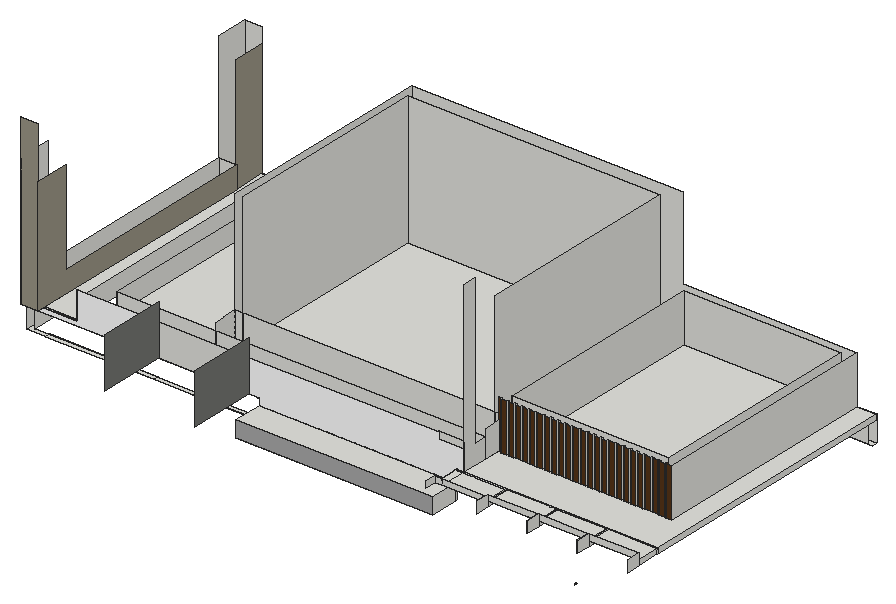
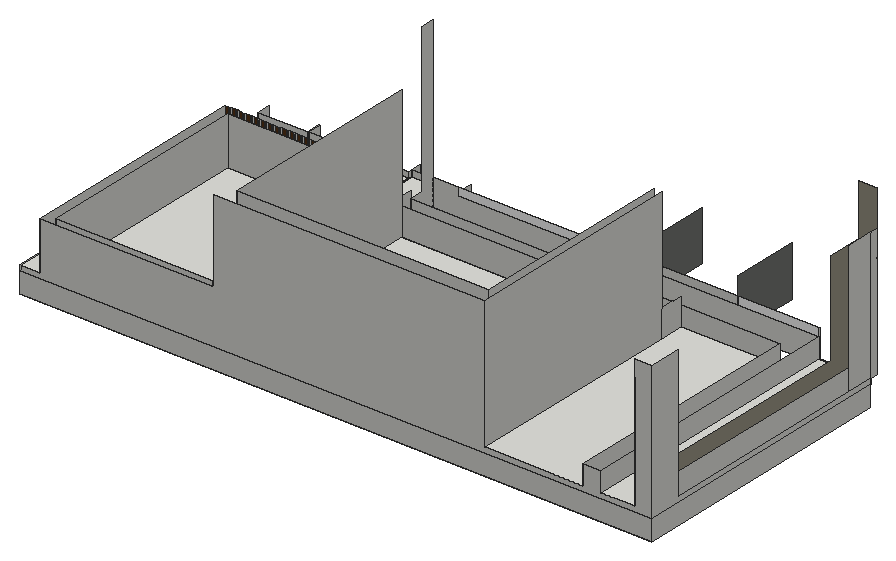
# SketchUp Ruby script. Lengths in inches.
U = 1.inch
M = Sketchup.active_model
def pt(a) = Geom::Point3d.new(a.map { |v| v * U })
def face(e, loops, mat)
  f = e.add_face(loops[0].map { |a| pt(a) })
  loops[1..].each { |l| e.add_face(l.map { |a| pt(a) }).erase! }
  f.material = f.back_material = mat if mat
  f
end
# faces: each face lists its corners as indices into pts; further lists are holes
def faces(e, pts, list, mat = nil) = list.each { |f| face(e, (f[0].is_a?(Array) ? f : [f]).map { |l| l.map { |i| pts[i] } }, mat) }
# xy, xz, yz: faces in a plane at the given z, y or x. An outline is a flat list of corners, or four numbers for a rectangle; further outlines are holes
def ring(l) = l.size == 4 ? [[l[0], l[1]], [l[2], l[1]], [l[2], l[3]], [l[0], l[3]]] : l.each_slice(2).to_a
def flat(e, list, mat, &to3) = list.each { |f| face(e, (f[0].is_a?(Array) ? f : [f]).map { |l| ring(l).map { |u, v| to3.(u, v) } }, mat) }
def xy(e, z, list, mat = nil) = flat(e, list, mat) { |x, y| [x, y, z] }
def xz(e, y, list, mat = nil) = flat(e, list, mat) { |x, z| [x, y, z] }
def yz(e, x, list, mat = nil) = flat(e, list, mat) { |y, z| [x, y, z] }
def lines(e, pts, list) = list.each { |a, b| e.add_line(pt(pts[a]), pt(pts[b])) }
# prism: a flat outline (further loops are holes) pulled along v
def prism(e, loops, v, mat = nil)
  f = face(e, loops, mat); d = Geom::Vector3d.new(v.map { |x| x * U })
  f.pushpull(f.normal.samedirection?(d) ? d.length : -d.length)
end
def box(e, o, s, mat = nil) = prism(e, [[o, [o[0] + s[0], o[1], o[2]], [o[0] + s[0], o[1] + s[1], o[2]], [o[0], o[1] + s[1], o[2]]]], [0, 0, s[2]], mat)
def at(x, y, z, deg = 0) = Geom::Transformation.translation(pt([x, y, z])) * Geom::Transformation.rotation(ORIGIN, Z_AXIS, deg.degrees)
def axes(o, x, y, z) = Geom::Transformation.new([*x, 0, *y, 0, *z, 0, *pt(o).to_a, 1])
def part(name) = M.definitions.add(name)
# library, detail: a bought-in or finely detailed component or shape, given as its bounding box
def library(name, o, s) = part(name).tap { |d| box(d.entities, o, s) }
def detail(e, o, s) = box(e.add_group.entities, o, s)
def put(e, d, t, mat = nil) = e.add_instance(d, t).tap { |i| i.material = mat if mat }
def group(e, t, mat = nil) = e.add_group.tap { |g| g.transformation = t; g.material = mat if mat }.entities
root = M.entities
M.materials.add("[0030_OldLace]").color = [86, 53, 24]
M.materials.add("[0128_White]").color = [255, 255, 255]
M.materials.add("[Color M03]").color = [170, 170, 170]
M.materials.add("[Concrete Tile]").color = [155, 150, 134]
M.materials.add("[Metal Seamed]").color = [116, 117, 113]
M.materials.add("[Wood Veneer 01]").color = [120, 70, 37]
xy(root,95.79,[[3323.99,846.1,3424.27,851.0625]])
xy(root,99.26,[[3261.3,810.97,3488.55,845.35]],"[Wood Veneer 01]")
xy(root,101.375,[[3184.99,845.35,3250.36,846.1],[2992.01,846.1,2992.01,1160.85,3720.76,1160.85,3720.76,1155.13,2997.72,1155.13,2997.72,851.0625,3184.99,851.0625,3184.99,846.1],[3184.99,846.1,3250.36,851.0625]])
xy(root,101.78,[[3014.67,845.35,3139.54,851.0625]])
xy(root,117.26,[[3261.3,810.97,3488.55,845.35]])
xy(root,125.1875,[[2992.01,845.35,3261.3,846.1]])
xy(root,131.1875,[[3488.55,814.22,3489.02,844.47],[3489.02,814.22,3496.96,844.47],[3496.96,814.22,3546.61,844.47],[3547.54,817.6,3604.66,844.47],[3605.72,817.6,3662.71,844.47],
  [3664.02,817.6,3720.76,844.47],[2992.01,837.03,3012.76,845.35],[3488.55,844.47,3489.02,845.35],[3489.02,844.47,3496.96,845.35],[3496.96,844.47,3720.76,846.1],
  [2992.01,845.35,3012.76,846.1],[3012.76,845.35,3050.93,846.1],[3488.55,845.35,3489.02,846.1],[3489.02,845.35,3496.96,846.1],[2992.01,846.1,3012.76,877.14],
  [3012.76,846.1,3050.93,846.1,3050.93,1160.85,3012.13,1160.85,3012.13,1122.97,3012.76,1122.97],[3496.96,846.1,3720.76,846.1,3720.76,1160.85,3698.33,1160.85,3698.33,893.65,3692.18,893.65,3692.18,895.71,3690.02,895.71,3690.02,893.65,3683.87,893.65,3683.87,895.71,3681.71,895.71,3681.71,894.34,3675.56,894.34,3675.56,895.71,3673.39,895.71,3673.39,894.34,3667.25,894.34,3667.25,895.71,3665.08,895.71,3665.08,894.34,3658.93,894.34,3658.93,895.71,3656.77,895.71,3656.77,894.34,3650.62,894.34,3650.62,895.71,3648.46,895.71,3648.46,894.34,3642.31,894.34,3642.31,895.71,3640.14,895.71,3640.14,894.34,3634,894.34,3634,895.71,3631.83,895.71,3631.83,894.34,3625.68,894.34,3625.68,895.71,3623.52,895.71,3623.52,894.34,3617.37,894.34,3617.37,895.71,3615.21,895.71,3615.21,894.34,3609.06,894.34,3609.06,895.71,3606.89,895.71,3606.89,894.34,3600.75,894.34,3600.75,895.71,3598.58,895.71,3598.58,894.34,3592.43,894.34,3592.43,895.71,3590.27,895.71,3590.27,894.34,3584.12,894.34,3584.12,895.71,3581.96,895.71,3581.96,894.34,3575.81,894.34,3575.81,895.71,3573.64,895.71,3573.64,894.34,3567.5,894.34,3567.5,895.71,3565.33,895.71,3565.33,894.34,3559.18,894.34,3559.18,895.71,3557.02,895.71,3557.02,894.34,3550.87,894.34,3550.87,895.71,3548.71,895.71,3548.71,894.34,3542.56,894.34,3542.56,895.71,3540.39,895.71,3540.39,894.34,3534.25,894.34,3534.25,895.71,3532.08,895.71,3532.08,894.34,3525.93,894.34,3525.93,895.71,3523.77,895.71,3523.77,894.34,3517.62,894.34,3517.62,895.71,3515.46,895.71,3515.46,894.34,3509.31,894.34,3509.31,895.71,3507.14,895.71,3507.14,894.34,3501,894.34,3501,895.71,3496.96,895.71],[2992.01,877.14,3012.76,1122.97],[3071.34,877.14,3184.99,1160.85],[3184.99,877.14,3496.96,905.7],
  [3505.43,904.18,3687.11,1152.375],[3194.375,905.7,3484.69,1143.26]])
xz(root,810.97,[[3261.3,99.26,3488.55,117.26]],"[Color M03]")
xz(root,814.22,[[3488.55,131.1875,3496.96,138.0625],[3496.96,131.1875,3546.61,138.0625]])
xz(root,817.6,[[3547.54,131.1875,3604.66,138.0625],[3605.72,131.1875,3662.71,138.0625],[3664.02,131.1875,3720.76,138.0625]])
xz(root,837.03,[[2992.01,131.1875,3012.76,324.5625]],"[Concrete Tile]")
xz(root,845.35,[[3261.3,99.26,3488.55,117.26],[3145.18,125.1875,3249.37,162.75]])
xz(root,845.35,[[3261.3,117.26,3488.55,117.26,3488.55,131.1875,3496.96,131.1875,3496.96,154.75,3467.75,154.75,3467.75,162.75,3249.37,162.75,3249.37,125.1875,3261.3,125.1875],[2992.01,125.1875,3145.18,125.1875,3145.18,162.75,3050.93,162.75,3050.93,131.1875,2992.01,131.1875]],"[0128_White]")
xz(root,846.1,[[2992.01,125.1875,2992.01,131.1875,3050.93,131.1875,3050.93,153.5625,3467.75,153.5625,3467.75,163,3496.96,163,3496.96,131.1875,3488.55,131.1875,3488.55,125.1875]])
xz(root,851.0625,[[3014.67,101.375,3139.54,101.78]])
xz(root,877.14,[[3071.34,131.1875,3184.99,153.5625],[3184.99,131.1875,3496.96,153.5625]])
xz(root,893.65,[[3683.87,131.1875,3690.02,186.75],[3692.18,131.1875,3698.33,186.75]],"[0030_OldLace]")
xz(root,894.34,[[3501,131.1875,3507.14,186.75],[3509.31,131.1875,3515.46,186.75],[3517.62,131.1875,3523.77,186.75],[3525.93,131.1875,3532.08,186.75],[3534.25,131.1875,3540.39,186.75],
  [3542.56,131.1875,3548.71,186.75],[3550.87,131.1875,3557.02,186.75],[3559.18,131.1875,3565.33,186.75],[3567.5,131.1875,3573.64,186.75],[3575.81,131.1875,3581.96,186.75],
  [3584.12,131.1875,3590.27,186.75],[3592.43,131.1875,3598.58,186.75],[3600.75,131.1875,3606.89,186.75],[3609.06,131.1875,3615.21,186.75],[3617.37,131.1875,3623.52,186.75],
  [3625.68,131.1875,3631.83,186.75],[3634,131.1875,3640.14,186.75],[3642.31,131.1875,3648.46,186.75],[3650.62,131.1875,3656.77,186.75],[3658.93,131.1875,3665.08,186.75],
  [3667.25,131.1875,3673.39,186.75],[3675.56,131.1875,3681.71,186.75]],"[0030_OldLace]")
xz(root,895.71,[[3496.96,131.1875,3501,186.75],[3507.14,131.1875,3509.31,186.75],[3515.46,131.1875,3517.62,186.75],[3523.77,131.1875,3525.93,186.75],[3532.08,131.1875,3534.25,186.75],
  [3540.39,131.1875,3542.56,186.75],[3548.71,131.1875,3550.87,186.75],[3557.02,131.1875,3559.18,186.75],[3565.33,131.1875,3567.5,186.75],[3573.64,131.1875,3575.81,186.75],
  [3581.96,131.1875,3584.12,186.75],[3590.27,131.1875,3592.43,186.75],[3598.58,131.1875,3600.75,186.75],[3606.89,131.1875,3609.06,186.75],[3615.21,131.1875,3617.37,186.75],
  [3623.52,131.1875,3625.68,186.75],[3631.83,131.1875,3634,186.75],[3640.14,131.1875,3642.31,186.75],[3648.46,131.1875,3650.62,186.75],[3656.77,131.1875,3658.93,186.75],
  [3665.08,131.1875,3667.25,186.75],[3673.39,131.1875,3675.56,186.75],[3681.71,131.1875,3683.87,186.75],[3690.02,131.1875,3692.18,186.75]],"[0030_OldLace]")
xz(root,904.18,[[3505.43,131.1875,3687.11,186.75]])
xz(root,905.7,[[3184.99,131.1875,3194.375,162.75],[3194.375,131.1875,3484.69,162.75],[3484.69,131.1875,3496.96,162.75]])
xz(root,1122.97,[[2992.01,131.1875,3012.13,156.5],[3012.13,131.1875,3012.76,156.5]])
xz(root,1143.26,[[3194.375,131.1875,3484.69,282.75]])
xz(root,1152.375,[[3505.43,131.1875,3687.11,186.75]])
xz(root,1155.13,[[2997.72,101.375,3715.04,125.1875]])
xz(root,1160.85,[[2992.01,101.375,3720.76,125.1875],[2992.01,125.1875,2992.01,282.75,3012.13,282.75,3012.13,131.1875,3050.93,131.1875,3050.93,153.5625,3071.34,153.5625,3071.34,131.1875,3184.99,131.1875,3184.99,282.75,3496.96,282.75,3496.96,186.75,3698.33,186.75,3698.33,131.1875,3720.76,131.1875,3720.76,125.1875]])
yz(root,2992.01,[[846.1,101.375,1160.85,125.1875],[845.35,125.1875,846.1,131.1875],[846.1,125.1875,846.1,131.1875,1122.97,131.1875,1122.97,282.75,1160.85,282.75,1160.85,125.1875],[837.03,131.1875,845.35,282.75],[845.35,131.1875,877.14,282.75],
  [877.14,131.1875,1122.97,156.5]])
yz(root,2997.72,[[851.0625,101.375,1155.13,125.1875]])
yz(root,3012.13,[[1122.97,131.1875,1160.85,264.75]],"[Concrete Tile]")
yz(root,3012.76,[[837.03,131.1875,1122.97,131.1875,1122.97,156.5,877.14,156.5,877.14,264.75,837.03,264.75]],"[Concrete Tile]")
yz(root,3050.93,[[845.35,131.1875,846.1,162.75],[846.1,131.1875,1160.85,153.5625]])
yz(root,3071.34,[[877.14,131.1875,1160.85,153.5625]])
yz(root,3145.18,[[767.72,125.1875,845.35,183.3125]],"[Metal Seamed]")
yz(root,3184.99,[[877.14,131.1875,877.14,162.125,888.95,162.125,888.95,162.75,905.7,162.75,905.7,131.1875],[905.7,131.1875,1160.85,282.75]])
yz(root,3194.375,[[905.7,131.1875,1143.26,282.75]])
yz(root,3249.37,[[767.72,125.1875,845.35,183.3125]],"[Metal Seamed]")
yz(root,3484.69,[[905.7,131.1875,1143.26,282.75]])
yz(root,3488.55,[[810.97,99.26,844.47,117.26],[844.47,99.26,845.35,117.26],[844.47,117.26,845.35,125.1875],[844.47,125.1875,845.35,131.1875],[845.35,125.1875,846.1,131.1875],
  [801.78,131.1875,814.22,138.0625]])
yz(root,3496.96,[[845.35,131.1875,846.1,163],[846.1,131.1875,877.14,131.1875,877.14,153.5625,861.24,153.5625,861.24,324.5625,846.1,324.5625],[877.14,131.1875,895.71,131.1875,895.71,162.75,890.39,162.75,890.39,162.125,877.14,162.125],[895.71,131.1875,905.7,162.75]])
yz(root,3501,[[894.34,131.1875,895.71,186.75]])
yz(root,3505.43,[[904.18,131.1875,905.7,186.75],[905.7,131.1875,1152.375,186.75]])
yz(root,3507.14,[[894.34,131.1875,895.71,186.75]])
yz(root,3509.31,[[894.34,131.1875,895.71,186.75]])
yz(root,3515.46,[[894.34,131.1875,895.71,186.75]])
yz(root,3517.62,[[894.34,131.1875,895.71,186.75]])
yz(root,3523.77,[[894.34,131.1875,895.71,186.75]])
yz(root,3525.93,[[894.34,131.1875,895.71,186.75]])
yz(root,3532.08,[[894.34,131.1875,895.71,186.75]])
yz(root,3534.25,[[894.34,131.1875,895.71,186.75]])
yz(root,3540.39,[[894.34,131.1875,895.71,186.75]])
yz(root,3542.56,[[894.34,131.1875,895.71,186.75]])
yz(root,3546.61,[[801.78,125.1875,814.22,138.0625],[814.22,125.1875,844.47,131.1875]])
yz(root,3547.54,[[801.78,125.1875,817.6,138.0625],[817.6,125.1875,844.47,131.1875]])
yz(root,3548.71,[[894.34,131.1875,895.71,186.75]])
yz(root,3550.87,[[894.34,131.1875,895.71,186.75]])
yz(root,3557.02,[[894.34,131.1875,895.71,186.75]])
yz(root,3559.18,[[894.34,131.1875,895.71,186.75]])
yz(root,3565.33,[[894.34,131.1875,895.71,186.75]])
yz(root,3567.5,[[894.34,131.1875,895.71,186.75]])
yz(root,3573.64,[[894.34,131.1875,895.71,186.75]])
yz(root,3575.81,[[894.34,131.1875,895.71,186.75]])
yz(root,3581.96,[[894.34,131.1875,895.71,186.75]])
yz(root,3584.12,[[894.34,131.1875,895.71,186.75]])
yz(root,3590.27,[[894.34,131.1875,895.71,186.75]])
yz(root,3592.43,[[894.34,131.1875,895.71,186.75]])
yz(root,3598.58,[[894.34,131.1875,895.71,186.75]])
yz(root,3600.75,[[894.34,131.1875,895.71,186.75]])
yz(root,3604.66,[[801.78,125.1875,817.6,138.0625],[817.6,125.1875,844.47,131.1875]])
yz(root,3605.72,[[801.78,125.1875,817.6,138.0625],[817.6,125.1875,844.47,131.1875]])
yz(root,3606.89,[[894.34,131.1875,895.71,186.75]])
yz(root,3609.06,[[894.34,131.1875,895.71,186.75]])
yz(root,3615.21,[[894.34,131.1875,895.71,186.75]])
yz(root,3617.37,[[894.34,131.1875,895.71,186.75]])
yz(root,3623.52,[[894.34,131.1875,895.71,186.75]])
yz(root,3625.68,[[894.34,131.1875,895.71,186.75]])
yz(root,3631.83,[[894.34,131.1875,895.71,186.75]])
yz(root,3634,[[894.34,131.1875,895.71,186.75]])
yz(root,3640.14,[[894.34,131.1875,895.71,186.75]])
yz(root,3642.31,[[894.34,131.1875,895.71,186.75]])
yz(root,3648.46,[[894.34,131.1875,895.71,186.75]])
yz(root,3650.62,[[894.34,131.1875,895.71,186.75]])
yz(root,3656.77,[[894.34,131.1875,895.71,186.75]])
yz(root,3658.93,[[894.34,131.1875,895.71,186.75]])
yz(root,3662.71,[[801.78,125.1875,817.6,138.0625],[817.6,125.1875,844.47,131.1875]])
yz(root,3664.02,[[801.78,125.1875,817.6,138.0625],[817.6,125.1875,844.47,131.1875]])
yz(root,3665.08,[[894.34,131.1875,895.71,186.75]])
yz(root,3667.25,[[894.34,131.1875,895.71,186.75]])
yz(root,3673.39,[[894.34,131.1875,895.71,186.75]])
yz(root,3675.56,[[894.34,131.1875,895.71,186.75]],"[0030_OldLace]")
yz(root,3681.71,[[894.34,131.1875,895.71,186.75]])
yz(root,3683.87,[[893.65,131.1875,895.71,186.75]],"[0030_OldLace]")
yz(root,3687.11,[[904.18,131.1875,1152.375,186.75]])
yz(root,3690.02,[[893.65,131.1875,895.71,186.75]])
yz(root,3692.18,[[893.65,131.1875,895.71,186.75]],"[0030_OldLace]")
yz(root,3698.33,[[893.65,131.1875,1160.85,186.75]])
yz(root,3720.76,[[801.78,125.1875,817.6,138.0625],[817.6,125.1875,844.47,131.1875],[844.47,125.1875,846.1,131.1875],[846.1,125.1875,1160.85,131.1875]])
p = [[3661.82,801.78,92.46],[3661.85,801.78,92.75],[3661.85,799.91,92.75],[3661.82,799.91,92.46],[3661.82,801.78,93.04],[3661.82,799.91,93.04],
  [3661.7,801.78,93.32],[3661.7,799.91,93.32]]
faces(root,p,[[0,1,2,3],[1,4,5,2],[4,6,7,5]])
